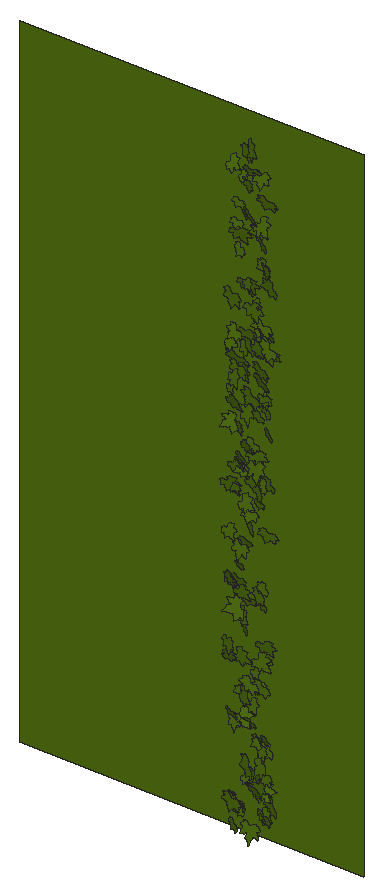
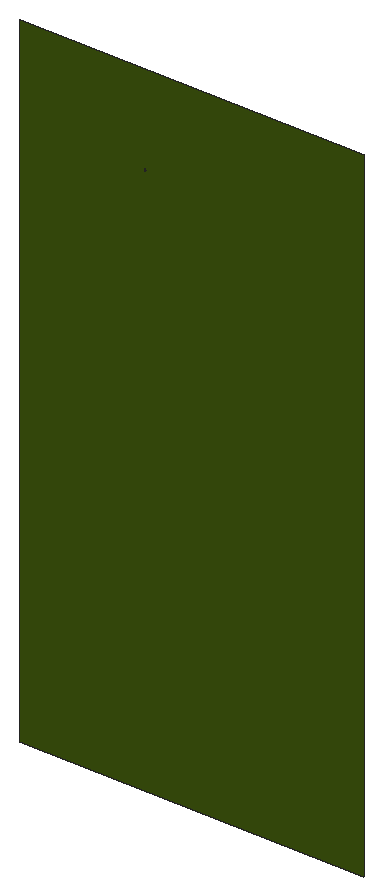
# SketchUp Ruby script. Lengths in inches.
U = 1.inch
M = Sketchup.active_model
def pt(a) = Geom::Point3d.new(a.map { |v| v * U })
def face(e, loops, mat)
  f = e.add_face(loops[0].map { |a| pt(a) })
  loops[1..].each { |l| e.add_face(l.map { |a| pt(a) }).erase! }
  f.material = f.back_material = mat if mat
  f
end
# faces: each face lists its corners as indices into pts; further lists are holes
def faces(e, pts, list, mat = nil) = list.each { |f| face(e, (f[0].is_a?(Array) ? f : [f]).map { |l| l.map { |i| pts[i] } }, mat) }
# xy, xz, yz: faces in a plane at the given z, y or x. An outline is a flat list of corners, or four numbers for a rectangle; further outlines are holes
def ring(l) = l.size == 4 ? [[l[0], l[1]], [l[2], l[1]], [l[2], l[3]], [l[0], l[3]]] : l.each_slice(2).to_a
def flat(e, list, mat, &to3) = list.each { |f| face(e, (f[0].is_a?(Array) ? f : [f]).map { |l| ring(l).map { |u, v| to3.(u, v) } }, mat) }
def xy(e, z, list, mat = nil) = flat(e, list, mat) { |x, y| [x, y, z] }
def xz(e, y, list, mat = nil) = flat(e, list, mat) { |x, z| [x, y, z] }
def yz(e, x, list, mat = nil) = flat(e, list, mat) { |y, z| [x, y, z] }
def lines(e, pts, list) = list.each { |a, b| e.add_line(pt(pts[a]), pt(pts[b])) }
# prism: a flat outline (further loops are holes) pulled along v
def prism(e, loops, v, mat = nil)
  f = face(e, loops, mat); d = Geom::Vector3d.new(v.map { |x| x * U })
  f.pushpull(f.normal.samedirection?(d) ? d.length : -d.length)
end
def box(e, o, s, mat = nil) = prism(e, [[o, [o[0] + s[0], o[1], o[2]], [o[0] + s[0], o[1] + s[1], o[2]], [o[0], o[1] + s[1], o[2]]]], [0, 0, s[2]], mat)
def at(x, y, z, deg = 0) = Geom::Transformation.translation(pt([x, y, z])) * Geom::Transformation.rotation(ORIGIN, Z_AXIS, deg.degrees)
def axes(o, x, y, z) = Geom::Transformation.new([*x, 0, *y, 0, *z, 0, *pt(o).to_a, 1])
def part(name) = M.definitions.add(name)
# library, detail: a bought-in or finely detailed component or shape, given as its bounding box
def library(name, o, s) = part(name).tap { |d| box(d.entities, o, s) }
def detail(e, o, s) = box(e.add_group.entities, o, s)
def put(e, d, t, mat = nil) = e.add_instance(d, t).tap { |i| i.material = mat if mat }
def group(e, t, mat = nil) = e.add_group.tap { |g| g.transformation = t; g.material = mat if mat }.entities
root = M.entities
M.materials.add("[Vegetation Blur 03]").color = [83, 114, 18]
c1 = part("ivy")
xy(c1.entities,0,[[0.782,0,0.786,0,0.787,0.005,0.789,0.009,0.821,0.072,0.875,0.147,1.001,0.272,1.073,0.331,1.137,0.363,1.178,0.379,1.223,0.384,1.272,0.383,1.311,0.374,1.36,0.355,1.399,0.334,1.491,0.285,1.541,0.244,1.583,0.199,1.617,0.15,1.64,0.128,1.662,0.115,1.717,0.105,1.745,0.093,1.784,0.054,1.819,0.057,1.854,0.064,1.882,0.075,1.896,0.074,1.91,0.071,1.937,0.063,1.964,0.053,1.99,0.038,2.016,0.015,2.034,0.002,2.04,0,2.038,0.003,2.036,0.007,2.033,0.038,2.036,0.068,2.045,0.1,2.055,0.116,2.064,0.123,2.077,0.129,2.088,0.129,2.106,0.132,2.118,0.13,2.179,0.132,2.207,0.133,2.225,0.133,2.242,0.138,2.22,0.162,2.207,0.186,2.206,0.213,2.212,0.236,2.228,0.262,2.247,0.274,2.298,0.283,2.355,0.294,2.37,0.296,2.376,0.295,2.377,0.3,2.377,0.303,2.385,0.329,2.411,0.37,2.426,0.392,2.449,0.407,2.511,0.426,2.561,0.444,2.619,0.466,2.589,0.469,2.561,0.476,2.501,0.5,2.449,0.516,2.424,0.523,2.401,0.535,2.377,0.556,2.372,0.568,2.36,0.575,2.268,0.586,2.225,0.592,2.207,0.599,2.194,0.61,2.143,0.65,2.13,0.664,2.122,0.682,2.123,0.7,2.13,0.719,2.148,0.75,2.17,0.781,2.195,0.807,2.221,0.828,2.284,0.874,2.291,0.88,2.288,0.887,2.276,0.9,2.267,0.916,2.265,0.933,2.273,0.967,2.292,1.002,2.313,1.03,2.334,1.054,2.348,1.067,2.358,1.074,2.363,1.076,2.362,1.081,2.35,1.094,2.347,1.11,2.35,1.143,2.359,1.18,2.385,1.254,2.415,1.324,2.448,1.393,2.45,1.4,2.446,1.398,2.44,1.394,2.427,1.383,2.402,1.36,2.376,1.339,2.345,1.324,2.305,1.309,2.282,1.303,2.273,1.306,2.245,1.294,2.212,1.287,2.187,1.291,2.163,1.301,2.142,1.316,2.134,1.327,2.124,1.325,2.09,1.292,2.053,1.259,2.014,1.234,1.973,1.215,1.954,1.21,1.931,1.208,1.909,1.212,1.893,1.22,1.879,1.233,1.872,1.248,1.867,1.281,1.864,1.319,1.821,1.258,1.773,1.197,1.726,1.141,1.698,1.121,1.679,1.116,1.666,1.117,1.647,1.122,1.632,1.129,1.62,1.141,1.617,1.154,1.617,1.219,1.621,1.254,1.623,1.268,1.623,1.281,1.618,1.314,1.606,1.346,1.603,1.375,1.607,1.403,1.603,1.467,1.599,1.499,1.605,1.525,1.614,1.552,1.629,1.577,1.635,1.589,1.629,1.587,1.618,1.582,1.596,1.566,1.581,1.556,1.568,1.552,1.557,1.55,1.545,1.553,1.531,1.562,1.522,1.572,1.504,1.591,1.486,1.611,1.474,1.631,1.457,1.666,1.455,1.684,1.457,1.698,1.452,1.715,1.444,1.728,1.424,1.754,1.419,1.772,1.423,1.786,1.434,1.819,1.444,1.848,1.446,1.855,1.44,1.861,1.43,1.867,1.386,1.904,1.349,1.948,1.326,1.973,1.31,1.995,1.288,2.048,1.284,2.153,1.287,2.254,1.284,2.255,1.282,2.253,1.278,2.247,1.274,2.237,1.266,2.216,1.226,2.125,1.208,2.076,1.184,2.033,1.155,1.984,1.135,1.942,1.111,1.899,1.083,1.861,1.053,1.85,1.059,1.83,1.061,1.809,1.056,1.79,1.049,1.767,1.04,1.749,1.018,1.733,0.994,1.726,0.942,1.734,0.95,1.6875,0.944,1.645,0.932,1.608,0.911,1.585,0.881,1.58,0.854,1.582,0.828,1.588,0.785,1.618,0.773,1.625,0.775,1.614,0.779,1.598,0.796,1.502,0.818,1.402,0.861,1.283,0.882,1.224,0.894,1.174,0.892,1.148,0.886,1.123,0.881,1.107,0.872,1.099,0.849,1.094,0.818,1.092,0.789,1.098,0.762,1.107,0.753,1.113,0.721,1.139,0.698,1.163,0.678,1.194,0.665,1.224,0.628,1.28,0.612,1.312,0.606,1.327,0.606,1.314,0.599,1.282,0.594,1.267,0.581,1.256,0.544,1.245,0.512,1.244,0.473,1.249,0.444,1.256,0.382,1.288,0.339,1.306,0.324,1.316,0.317,1.324,0.309,1.326,0.27,1.314,0.227,1.313,0.185,1.3125,0.152,1.317,0.122,1.328,0.092,1.345,0.073,1.353,0.079,1.338,0.092,1.308,0.117,1.249,0.13,1.215,0.139,1.164,0.147,1.148,0.157,1.136,0.163,1.122,0.174,1.086,0.177,1.067,0.182,1.054,0.186,1.043,0.191,1.038,0.211,1.028,0.237,1.005,0.25,0.974,0.253,0.96,0.25,0.944,0.242,0.914,0.243,0.906,0.249,0.902,0.26,0.894,0.289,0.88,0.307,0.873,0.322,0.862,0.364,0.799,0.403,0.738,0.431,0.709,0.439,0.691,0.441,0.678,0.4375,0.66,0.428,0.645,0.394,0.623,0.303,0.594,0.255,0.581,0.214,0.577,0.179,0.573,0.173,0.568,0.175,0.561,0.167,0.55,0.141,0.523,0.113,0.503,0.077,0.49,0.045,0.486,0.026,0.485,0.019,0.486,0.011,0.483,0,0.471,0.014,0.467,0.044,0.455,0.058,0.447,0.07,0.438,0.097,0.411,0.125,0.394,0.158,0.377,0.174,0.366,0.182,0.359,0.185,0.361,0.242,0.331,0.253,0.316,0.258,0.303,0.262,0.283,0.274,0.278,0.308,0.274,0.341,0.252,0.366,0.226,0.366,0.222,0.37,0.22,0.38,0.221,0.395,0.221,0.425,0.216,0.45,0.207,0.465,0.192,0.473,0.178,0.484,0.15,0.489,0.116,0.483,0.089,0.468,0.058,0.45,0.035,0.435,0.018,0.429,0.011,0.434,0.012,0.438,0.014,0.469,0.019,0.542,0.016,0.581,0.015,0.612,0.027,0.68,0.055,0.696,0.057,0.712,0.052,0.73,0.045,0.741,0.036,0.766,0.014]])
xz(root,174.6,[[113.54,5,138,51]],"[Vegetation Blur 03]")
put(root,c1,axes([128.65,173.8,21.06],[0.25004,-0.05522,0.19659],[0.24228,0.07618,-0.20189],[0.00655,-0.71038,-0.03693]),"[Vegetation Blur 03]")
put(root,c1,axes([129.15,173.8,7.81],[0.43018,0.03461,-0.33433],[-0.40999,0.03807,-0.35076],[-0.00059,-1.2218,-0.0204]),"[Vegetation Blur 03]")
put(root,c1,axes([128.58,173.8,16.03],[0.13975,-0.17275,0.35559],[0.44281,0.11446,-0.10717],[0.0284,-0.9346,-0.07885]),"[Vegetation Blur 03]")
put(root,c1,axes([128.4,173.8,24.2],[0.35229,-0.00554,0.29733],[0.36145,-0.12544,-0.28562],[-0.04568,-1.0353,0.03302]),"[Vegetation Blur 03]")
put(root,c1,axes([129.33,173.8,32.11],[0.3559,-0.06669,-0.38571],[-0.47242,-0.14005,-0.28653],[0.03508,-1.20938,0.05445]),"[Vegetation Blur 03]")
put(root,c1,axes([128.67,173.8,7.72],[0.62299,-0.15418,-0.12642],[-0.15294,0.05244,-0.51207],[-0.07884,-1.31998,-0.00558]),"[Vegetation Blur 03]")
put(root,c1,axes([128.64,173.8,35.97],[0.08788,0.15958,0.41108],[0.50211,-0.20702,-0.05886],[-0.08717,-1.03158,0.0754]),"[Vegetation Blur 03]")
put(root,c1,axes([128.24,173.8,27.21],[0.49372,-0.08066,0.3359],[0.41334,0.06825,-0.4021],[-0.00879,-1.32093,-0.04129]),"[Vegetation Blur 03]")
put(root,c1,axes([129.14,173.8,6.14],[0.34936,-0.1754,-0.17065],[-0.20005,0.12722,-0.29335],[-0.10473,-0.82812,-0.00892]),"[Vegetation Blur 03]")
put(root,c1,axes([128.96,173.8,27.82],[0.46927,-0.11869,-0.14311],[-0.17217,0.07416,-0.3857],[-0.06659,-1.02821,-0.0113]),"[Vegetation Blur 03]")
put(root,c1,axes([128.82,173.8,33.45],[0.20111,-0.0492,0.23305],[0.27447,-0.17313,-0.16352],[-0.08231,-0.69755,0.02415]),"[Vegetation Blur 03]")
put(root,c1,axes([128.55,173.8,17.51],[0.49387,-0.24848,0.14861],[0.17062,-0.13992,-0.41447],[-0.13648,-1.07408,0.01961]),"[Vegetation Blur 03]")
put(root,c1,axes([128.875,173.8,35.9375],[0.61818,0.02753,-0.20694],[-0.25253,0.20999,-0.49806],[-0.0265,-1.35881,-0.08116]),"[Vegetation Blur 03]")
put(root,c1,axes([128.74,173.8,47.34],[0.1221,0.15901,0.36769],[0.45566,-0.11863,-0.09271],[-0.03634,-0.95319,0.07288]),"[Vegetation Blur 03]")
put(root,c1,axes([129.03,173.8,7.77],[0.53938,-0.11783,-0.24861],[-0.28048,0.34993,-0.43141],[-0.13192,-1.22575,-0.09926]),"[Vegetation Blur 03]")
put(root,c1,axes([128.75,173.8,13.0625],[0.49941,-0.26714,0.04177],[0.06827,0.12648,-0.4165],[-0.1217,-1.02529,-0.06226]),"[Vegetation Blur 03]")
put(root,c1,axes([129.9375,173.8,45.38],[0.10747,0.09693,-0.42949],[-0.50045,0.37307,-0.07017],[-0.16944,-1.0404,-0.06517]),"[Vegetation Blur 03]")
put(root,c1,axes([128.73,173.8,39.95],[0.66254,-0.24066,-0.04091],[-0.05165,-0.00895,-0.54898],[-0.11628,-1.36725,0.01079]),"[Vegetation Blur 03]")
put(root,c1,axes([128.66,173.8,21.45],[0.34584,-0.27967,0.31588],[0.38688,-0.124,-0.2994],[-0.13639,-1.06088,-0.04828]),"[Vegetation Blur 03]")
put(root,c1,axes([129.34,173.8,37.8],[0.41213,-0.1677,-0.21359],[-0.27008,-0.08234,-0.33694],[-0.04682,-1.00125,0.06348]),"[Vegetation Blur 03]")
put(root,c1,axes([129.83,173.8,20.5],[0.32603,-0.13943,-0.47145],[-0.58131,-0.12239,-0.26207],[0.01889,-1.35947,0.07195]),"[Vegetation Blur 03]")
put(root,c1,axes([129.27,173.8,44.4],[0.32282,0.01218,-0.05233],[-0.06347,-0.05325,-0.26277],[0.01083,-0.67519,0.01978]),"[Vegetation Blur 03]")
put(root,c1,axes([128.86,173.8,28.54],[0.35919,-0.07581,0.24051],[0.29623,0.02355,-0.29351],[-0.02119,-0.9558,-0.02631]),"[Vegetation Blur 03]")
put(root,c1,axes([129.44,173.8,45.8],[0.32239,-0.01176,-0.10948],[-0.13423,-0.01041,-0.2631],[-0.00333,-0.71849,0.00561]),"[Vegetation Blur 03]")
put(root,c1,axes([129.96,173.8,7.01],[0.06839,0.01536,-0.24268],[-0.29667,-0.04173,-0.0561],[0.02144,-0.62648,-0.00221]),"[Vegetation Blur 03]")
put(root,c1,axes([129.86,173.8,14.71],[0.15181,-0.00524,-0.23084],[-0.28286,-0.00517,-0.12389],[0.00101,-0.66057,0.0028]),"[Vegetation Blur 03]")
put(root,c1,axes([128.75,173.8,32.62],[0.38193,-0.25872,0.35613],[0.44798,0.02235,-0.31745],[-0.07443,-1.19311,-0.08317]),"[Vegetation Blur 03]")
put(root,c1,axes([130.19,173.8,18.9],[0.06026,0.01776,-0.40154],[-0.46093,0.35917,-0.04358],[-0.17229,-0.95467,-0.02387]),"[Vegetation Blur 03]")
put(root,c1,axes([129.62,173.8,29.6],[0.28037,-0.06157,-0.15463],[-0.18018,0.15229,-0.22714],[-0.06579,-0.67947,-0.0369]),"[Vegetation Blur 03]")
put(root,c1,axes([128.92,173.8,34.13],[0.31073,-0.06738,0.37222],[0.4328,-0.32267,-0.24985],[-0.14749,-1.08882,0.05101]),"[Vegetation Blur 03]")
put(root,c1,axes([129.22,173.8,21.7],[0.47998,-0.11829,-0.01678],[-0.01365,0.11877,-0.39191],[-0.0595,-0.98146,-0.0454]),"[Vegetation Blur 03]")
put(root,c1,axes([129.05,173.8,12.68],[0.45593,-0.14871,0.15697],[0.17169,-0.25336,-0.36992],[-0.11285,-0.98625,0.07136]),"[Vegetation Blur 03]")
put(root,c1,axes([129.45,173.8,22.55],[0.3065,-0.10801,0.00878],[0.01921,0.10156,-0.25024],[-0.05001,-0.62289,-0.04232]),"[Vegetation Blur 03]")
put(root,c1,axes([129.17,173.8,35.42],[0.63233,-0.20373,-0.05495],[-0.06893,-0.01048,-0.5222],[-0.0979,-1.30853,0.01274]),"[Vegetation Blur 03]")
put(root,c1,axes([128.9,173.8,43.53],[0.56255,-0.01811,0.20546],[0.25121,0.13405,-0.45628],[0.01862,-1.26114,-0.05145]),"[Vegetation Blur 03]")
put(root,c1,axes([130.03,173.8,28.98],[0.19807,-0.04882,-0.25327],[-0.31096,-0.06252,-0.16009],[0.01294,-0.755,0.02963]),"[Vegetation Blur 03]")
put(root,c1,axes([129.4,173.8,29.22],[0.42582,-0.25778,-0.01572],[0.00049,0.14225,-0.35818],[-0.12674,-0.86554,-0.05419]),"[Vegetation Blur 03]")
put(root,c1,axes([129.91,173.8,24.24],[0.26692,0.10027,-0.19485],[-0.24358,0.09015,-0.21495],[0.00657,-0.73139,-0.05321]),"[Vegetation Blur 03]")
put(root,c1,axes([129.65,173.8,43.04],[0.38208,-0.19358,-0.10183],[-0.13229,-0.03969,-0.31874],[-0.08317,-0.82615,0.03917]),"[Vegetation Blur 03]")
put(root,c1,axes([128.96,173.8,12.34],[0.39393,0.1891,0.39235],[0.48905,-0.10099,-0.3194],[0.01969,-1.27498,0.08349]),"[Vegetation Blur 03]")
put(root,c1,axes([129.36,173.8,31.4375],[0.37901,-0.24998,0.16924],[0.20826,-0.05609,-0.32368],[-0.11995,-0.88726,-0.02722]),"[Vegetation Blur 03]")
put(root,c1,axes([129.39,173.8,34.7],[0.23197,-0.0436,0.29061],[0.3566,0.00644,-0.18945],[-0.00894,-0.8745,-0.01588]),"[Vegetation Blur 03]")
put(root,c1,axes([130.34,173.8,10.44],[0.28462,-0.17247,-0.45638],[-0.54186,0.28495,-0.24203],[-0.16158,-1.25936,0.00774]),"[Vegetation Blur 03]")
put(root,c1,axes([129.36,173.8,23.98],[0.58607,-0.17658,0.01299],[0.00501,-0.15402,-0.47969],[-0.08713,-1.19658,0.05983]),"[Vegetation Blur 03]")
put(root,c1,axes([129.2,173.8,20.58],[0.39343,-0.07208,0.30532],[0.37571,0.06003,-0.32024],[-0.0052,-1.11557,-0.03696]),"[Vegetation Blur 03]")
put(root,c1,axes([129.69,173.8,46.95],[0.0888,0.09674,0.25308],[0.31076,-0.1168,-0.0656],[-0.0424,-0.6534,0.0492]),"[Vegetation Blur 03]")
put(root,c1,axes([130.12,173.8,36.92],[0.29115,-0.21346,-0.2217],[-0.27097,0.0878,-0.25032],[-0.10549,-0.81469,0.03111]),"[Vegetation Blur 03]")
put(root,c1,axes([130.64,173.8,29.1],[0.14596,0.116,-0.44941],[-0.55223,-0.05004,-0.12149],[0.03805,-1.17121,-0.03932]),"[Vegetation Blur 03]")
put(root,c1,axes([129.37,173.8,16.21],[0.18573,-0.07263,0.44986],[0.55141,-0.04477,-0.15278],[-0.03192,-1.19609,-0.0216]),"[Vegetation Blur 03]")
put(root,c1,axes([129.875,173.8,20.51],[0.38415,0.08832,-0.09325],[-0.11924,0.10565,-0.31143],[0.02608,-0.81794,-0.0503]),"[Vegetation Blur 03]")
put(root,c1,axes([130.125,173.8,45.38],[0.42548,-0.09437,-0.33716],[-0.38139,0.39508,-0.33797],[-0.16527,-1.15464,-0.08808]),"[Vegetation Blur 03]")
put(root,c1,axes([130.2,173.8,49.45],[0.35368,-0.15187,-0.29343],[-0.34945,0.17479,-0.29479],[-0.11221,-1.02299,-0.00681]),"[Vegetation Blur 03]")
put(root,c1,axes([130.3125,173.8,12.8],[0.21856,0.08137,-0.22546],[-0.27868,0.10188,-0.17416],[-0.01478,-0.71768,-0.05028]),"[Vegetation Blur 03]")
put(root,c1,axes([129.79,173.8,8.72],[0.17985,0.03398,0.21034],[0.25744,-0.07475,-0.14472],[-0.02044,-0.64238,0.02797]),"[Vegetation Blur 03]")
put(root,c1,axes([130.29,173.8,37.11],[0.38374,-0.03816,-0.34105],[-0.41282,0.15382,-0.31209],[-0.06752,-1.15732,-0.03024]),"[Vegetation Blur 03]")
put(root,c1,axes([130.66,173.8,25.25],[0.07886,-0.02245,-0.3122],[-0.36365,0.24601,-0.06396],[-0.11923,-0.76517,-0.0114]),"[Vegetation Blur 03]")
put(root,c1,axes([129.59,173.8,25.98],[0.16307,0.08475,0.41488],[0.5096,-0.07153,-0.13111],[-0.02064,-1.09626,0.04063]),"[Vegetation Blur 03]")
put(root,c1,axes([130.22,173.8,15.56],[0.42678,-0.01115,-0.26433],[-0.32354,-0.0687,-0.34749],[0.01587,-1.10035,0.02437]),"[Vegetation Blur 03]")
put(root,c1,axes([129.66,173.8,18.98],[0.16191,-0.03187,0.41572],[0.48687,-0.31523,-0.1301],[-0.15054,-1.05373,0.02635]),"[Vegetation Blur 03]")
put(root,c1,axes([129.61,173.8,37.48],[0.51847,-0.08238,0.09913],[0.12469,0.09368,-0.42215],[-0.02842,-1.09178,-0.0437]),"[Vegetation Blur 03]")
put(root,c1,axes([129.42,173.8,40.53],[0.5764,-0.04158,0.19028],[0.23362,0.17732,-0.46527],[0.01378,-1.26714,-0.07135]),"[Vegetation Blur 03]")
put(root,c1,axes([129.62,173.8,34.95],[0.39018,-0.19806,0.28181],[0.33951,-0.13277,-0.32778],[-0.115,-1.06391,-0.01155]),"[Vegetation Blur 03]")
put(root,c1,axes([129.76,173.8,13.8125],[0.12637,-0.06641,0.44261],[0.52763,-0.25805,-0.10643],[-0.12947,-1.11645,-0.00173]),"[Vegetation Blur 03]")
put(root,c1,axes([130.27,173.8,40.41],[0.29856,-0.10941,-0.11062],[-0.12269,0.1536,-0.24445],[-0.0784,-0.65702,-0.03873]),"[Vegetation Blur 03]")
put(root,c1,axes([130.22,173.8,34.02],[0.54012,-0.12372,-0.29412],[-0.3556,0.12595,-0.44329],[-0.0839,-1.33021,-0.01462]),"[Vegetation Blur 03]")
put(root,c1,axes([130.06,173.8,26.15],[0.44019,0.01869,-0.05575],[-0.06711,-0.08998,-0.3577],[0.01564,-0.91223,0.03414]),"[Vegetation Blur 03]")
put(root,c1,axes([129.83,173.8,30.07],[0.25746,-0.20708,0.31713],[0.39391,-0.05224,-0.21837],[-0.07715,-0.95777,-0.05666]),"[Vegetation Blur 03]")
put(root,c1,axes([129.96,173.8,47.22],[0.42985,-0.21428,0.06487],[0.08397,0.02008,-0.36019],[-0.10055,-0.89931,-0.0235]),"[Vegetation Blur 03]")
put(root,c1,axes([129.98,173.8,40.5],[0.26598,-0.07146,0.22657],[0.27016,-0.13937,-0.21816],[-0.07275,-0.7788,0.01825]),"[Vegetation Blur 03]")
put(root,c1,axes([130.51,173.8,30.82],[0.32974,-0.02071,-0.22461],[-0.27537,-0.01528,-0.26905],[-0.00296,-0.88368,0.00992]),"[Vegetation Blur 03]")
put(root,c1,axes([129.77,173.8,32.55],[0.51632,-0.17161,0.26126],[0.29868,-0.283,-0.42241],[-0.14219,-1.21766,0.06135]),"[Vegetation Blur 03]")
put(root,c1,axes([129.91,173.8,6.21],[0.65317,-0.15035,0.08957],[0.09783,-0.2124,-0.5313],[-0.08838,-1.34629,0.07382]),"[Vegetation Blur 03]")
put(root,c1,axes([131.09,173.8,32.67],[0.16409,0.0678,-0.30247],[-0.37206,0.03564,-0.13319],[-0.00256,-0.83328,-0.0303]),"[Vegetation Blur 03]")
put(root,c1,axes([130.08,173.8,27.74],[0.26787,-0.06927,0.33281],[0.40897,0.07748,-0.21671],[0.01312,-1.00101,-0.0398]),"[Vegetation Blur 03]")
put(root,c1,axes([129.9375,173.8,47.96],[0.62307,-0.149,0.09151],[0.12235,0.19755,-0.50432],[-0.05332,-1.28769,-0.08796]),"[Vegetation Blur 03]")
put(root,c1,axes([131,173.8,11.95],[0.28434,-0.07307,-0.35446],[-0.41994,0.239,-0.23213],[-0.11635,-1.04116,-0.02841]),"[Vegetation Blur 03]")
put(root,c1,axes([131.1,173.8,44.49],[0.19509,-0.01615,-0.32843],[-0.40182,0.04546,-0.15934],[-0.0233,-0.91916,-0.00211]),"[Vegetation Blur 03]")
put(root,c1,axes([130.15,173.8,8.75],[0.57489,-0.26657,0.03866],[0.06843,0.18847,-0.47339],[-0.11976,-1.17196,-0.08492]),"[Vegetation Blur 03]")
put(root,c1,axes([131.05,173.8,28.49],[0.3874,-0.28987,-0.42046],[-0.49062,0.32448,-0.33628],[-0.21109,-1.28615,0.00992]),"[Vegetation Blur 03]")
put(root,c1,axes([130.21,173.8,13.6875],[0.31135,-0.03304,0.2876],[0.34314,-0.19604,-0.25097],[-0.08184,-0.94759,0.04189]),"[Vegetation Blur 03]")
put(root,c1,axes([131.08,173.8,11.82],[0.20749,-0.03484,-0.23563],[-0.28917,-0.01288,-0.16931],[-0.00479,-0.73151,0.0142]),"[Vegetation Blur 03]")
put(root,c1,axes([130.3,173.8,48.75],[0.0835,-0.00667,0.46395],[0.54474,-0.33722,-0.06606],[-0.16259,-1.13325,0.01693]),"[Vegetation Blur 03]")
put(root,c1,axes([129.97,173.8,39.15],[0.58643,-0.10608,0.2337],[0.28408,-0.0778,-0.48036],[-0.06289,-1.34069,0.00938]),"[Vegetation Blur 03]")
put(root,c1,axes([130.09,173.8,29.65],[0.54429,0.0275,0.19656],[0.23996,0.06284,-0.44397],[0.02457,-1.22318,-0.01839]),"[Vegetation Blur 03]")
put(root,c1,axes([130.53,173.8,15.82],[0.22624,-0.03067,0.2044],[0.24637,-0.10398,-0.18409],[-0.04741,-0.6867,0.01875]),"[Vegetation Blur 03]")
put(root,c1,axes([131.44,173.8,20.83],[0.12874,0.00958,-0.35889],[-0.43298,0.16781,-0.10275],[-0.07698,-0.92784,-0.02229]),"[Vegetation Blur 03]")
put(root,c1,axes([130.94,173.8,35.04],[0.44147,-0.0788,-0.2903],[-0.33877,0.28169,-0.35517],[-0.11502,-1.13213,-0.06817]),"[Vegetation Blur 03]")
put(root,c1,axes([131.13,173.8,9.77],[0.29889,-0.0519,-0.2268],[-0.27904,-0.05258,-0.24304],[-0.001,-0.83818,0.02929]),"[Vegetation Blur 03]")
put(root,c1,axes([130.71,173.8,39.43],[0.18943,-0.02258,0.18927],[0.22327,-0.15119,-0.15168],[-0.06367,-0.59736,0.03124]),"[Vegetation Blur 03]")
put(root,c1,axes([130.37,173.8,9.71],[0.48095,-0.24511,0.14889],[0.18901,0.01686,-0.4023],[-0.10837,-1.05836,-0.04089]),"[Vegetation Blur 03]")
put(root,c1,axes([130.86,173.8,26.97],[0.32248,-0.05987,-0.04087],[-0.04757,0.05862,-0.26354],[-0.03303,-0.669,-0.01944]),"[Vegetation Blur 03]")
put(root,c1,axes([130.92,173.8,38.23],[0.34481,-0.20074,-0.10306],[-0.10927,0.15385,-0.29065],[-0.11628,-0.7398,-0.03248]),"[Vegetation Blur 03]")
put(root,c1,axes([130.96,173.8,15.59],[0.47072,-0.03676,-0.23219],[-0.28418,0.02801,-0.38445],[-0.02233,-1.13149,-0.00197]),"[Vegetation Blur 03]")
put(root,c1,axes([131.53,173.8,21.86],[0.16539,-0.02327,-0.29289],[-0.35869,0.02592,-0.13523],[-0.01618,-0.81273,0.00407]),"[Vegetation Blur 03]")
put(root,c1,axes([130.79,173.8,35.81],[0.56634,-0.19077,-0.13861],[-0.15859,0.16167,-0.4666],[-0.11086,-1.2059,-0.04063]),"[Vegetation Blur 03]")
put(root,c1,axes([130.82,173.8,14.78],[0.17104,0.07406,0.23051],[0.28468,-0.03259,-0.13906],[0.00499,-0.6787,0.03183]),"[Vegetation Blur 03]")
put(root,c1,axes([130.81,173.8,21.41],[0.49502,-0.2424,-0.04719],[-0.06027,-0.00753,-0.41504],[-0.11656,-1.02555,0.0142]),"[Vegetation Blur 03]")
put(root,c1,axes([130.33,173.8,29.15],[0.58365,-0.1286,0.23072],[0.26562,-0.28309,-0.47237],[-0.11521,-1.30414,0.07979]),"[Vegetation Blur 03]")
put(root,c1,axes([130.93,173.8,38.5625],[0.53942,-0.03341,-0.15907],[-0.19556,-0.07489,-0.43924],[-0.00287,-1.17788,0.03244]),"[Vegetation Blur 03]")
put(root,c1,axes([130.52,173.8,36.5],[0.30631,-0.15054,0.36025],[0.43855,-0.11732,-0.25607],[-0.08874,-1.09937,-0.022]),"[Vegetation Blur 03]")
put(root,c1,axes([131.67,173.8,28.4375],[0.12105,-0.13191,-0.28197],[-0.3442,0.10689,-0.10629],[-0.07075,-0.74572,0.03464]),"[Vegetation Blur 03]")
put(root,c1,axes([130.57,173.8,8.97],[0.52242,-0.17809,0.13316],[0.16214,-0.04009,-0.43214],[-0.08844,-1.12553,-0.00568]),"[Vegetation Blur 03]")
put(root,c1,axes([131.51,173.8,42.55],[0.26106,-0.06742,-0.29363],[-0.35973,0.03582,-0.21432],[-0.03335,-0.91402,0.01326]),"[Vegetation Blur 03]")
put(root,c1,axes([131.14,173.8,43.82],[0.38591,-0.21569,-0.14541],[-0.15737,0.19687,-0.32414],[-0.13402,-0.85224,-0.03808]),"[Vegetation Blur 03]")
put(root,c1,axes([131.84,173.8,28.625],[0.1471,0.09742,-0.39347],[-0.48397,0.0748,-0.1176],[-0.02114,-1.03455,-0.04555]),"[Vegetation Blur 03]")
put(root,c1,axes([130.49,173.8,16.35],[0.3582,0.03063,0.42978],[0.52659,-0.05959,-0.29166],[-0.01559,-1.30923,0.02333]),"[Vegetation Blur 03]")
put(root,c1,axes([130.84,173.8,16.62],[0.36162,0.06548,0.17991],[0.22033,0.0215,-0.29621],[0.03262,-0.87124,0.00621]),"[Vegetation Blur 03]")
put(root,c1,axes([131.63,173.8,37.49],[0.37878,0.01189,-0.41383],[-0.50562,-0.09055,-0.30867],[0.03871,-1.29927,0.01773]),"[Vegetation Blur 03]")
put(root,c1,axes([131.15,173.8,46.52],[0.51764,0.02568,-0.18283],[-0.22378,0.14257,-0.41887],[-0.01616,-1.15189,-0.05592]),"[Vegetation Blur 03]")
put(root,c1,axes([131.08,173.8,7.34],[0.50401,-0.18357,-0.11952],[-0.1351,0.15116,-0.41597],[-0.10561,-1.06941,-0.03828]),"[Vegetation Blur 03]")
put(root,c1,axes([130.79,173.8,47.9375],[0.54024,-0.08088,0.09089],[0.10321,-0.19815,-0.43637],[-0.05739,-1.11765,0.07079]),"[Vegetation Blur 03]")
put(root,c1,axes([130.68,173.8,8.1],[0.37101,0.18964,0.31894],[0.39968,-0.06988,-0.30314],[0.03834,-1.10666,0.0738]),"[Vegetation Blur 03]")
put(root,c1,axes([132.01,173.8,41.29],[0.18125,0.04011,-0.45454],[-0.55361,0.15105,-0.14494],[-0.06386,-1.19573,-0.03356]),"[Vegetation Blur 03]")
put(root,c1,axes([131.61,173.8,33.625],[0.34504,-0.21965,-0.31495],[-0.37042,0.22285,-0.29474],[-0.152,-1.04167,0.00335]),"[Vegetation Blur 03]")
put(root,c1,axes([131.85,173.8,11.85],[0.21313,-0.07118,-0.35531],[-0.43534,0.04461,-0.17534],[-0.03471,-0.99647,0.01753]),"[Vegetation Blur 03]")
put(root,c1,axes([130.66,173.8,44.22],[0.34036,0.06769,0.40355],[0.48921,-0.24292,-0.26842],[-0.07909,-1.21115,0.07639]),"[Vegetation Blur 03]")
put(root,c1,axes([131.16,173.8,9.97],[0.51001,-0.14732,-0.08686],[-0.10909,-0.02593,-0.41973],[-0.06746,-1.07179,0.02209]),"[Vegetation Blur 03]")
put(root,c1,axes([131.66,173.8,38.11],[0.28115,-0.04858,-0.24392],[-0.28246,0.2397,-0.22437],[-0.10049,-0.80964,-0.05179]),"[Vegetation Blur 03]")
put(root,c1,axes([131.26,173.8,25.31],[0.48743,0.04761,-0.1367],[-0.16843,0.04371,-0.39762],[0.01495,-1.05971,-0.02254]),"[Vegetation Blur 03]")
put(root,c1,axes([131.69,173.8,31.74],[0.24639,-0.0769,-0.23479],[-0.27054,0.21951,-0.20041],[-0.10474,-0.7479,-0.03468]),"[Vegetation Blur 03]")
put(root,c1,axes([131.04,173.8,11.01],[0.30019,-0.07683,0.21744],[0.25164,-0.21034,-0.24309],[-0.09515,-0.7987,0.0431]),"[Vegetation Blur 03]")
put(root,c1,axes([131.98,173.8,8.45],[0.27997,-0.09905,-0.45822],[-0.54252,0.30141,-0.23104],[-0.15235,-1.25535,-0.01932]),"[Vegetation Blur 03]")
put(root,c1,axes([131.23,173.8,11.01],[0.55698,-0.45746,-0.14027],[-0.2006,-0.09744,-0.48055],[-0.19678,-1.19551,0.09284]),"[Vegetation Blur 03]")
put(root,c1,axes([130.84,173.8,36.5],[0.59787,0.07047,0.08314],[0.09735,0.14687,-0.48587],[0.04553,-1.23935,-0.05285]),"[Vegetation Blur 03]")
put(root,c1,axes([131.32,173.8,33.21],[0.05918,0.07636,0.27369],[0.32495,-0.20144,-0.03796],[-0.0908,-0.67116,0.04253]),"[Vegetation Blur 03]")
put(root,c1,axes([130.79,173.8,17.73],[0.50143,-0.04661,0.23263],[0.28578,0.12116,-0.40648],[0.00953,-1.18071,-0.05089]),"[Vegetation Blur 03]")
put(root,c1,axes([131.03,173.8,33.69],[0.45211,-0.0957,0.11404],[0.13937,-0.02195,-0.37092],[-0.04759,-0.97354,-0.00285]),"[Vegetation Blur 03]")
put(root,c1,axes([131.25,173.8,11.97],[0.28812,-0.17967,0.12477],[0.15963,0.01216,-0.24278],[-0.07425,-0.67108,-0.0378]),"[Vegetation Blur 03]")
put(root,c1,axes([131.26,173.8,42.25],[0.44121,-0.22953,-0.01023],[-0.00431,0.06987,-0.3705],[-0.11216,-0.9056,-0.026]),"[Vegetation Blur 03]")
put(root,c1,axes([131.12,173.8,6.72],[0.18512,0.00647,0.33943],[0.41367,-0.0999,-0.14998],[-0.04308,-0.93144,0.01844]),"[Vegetation Blur 03]")
